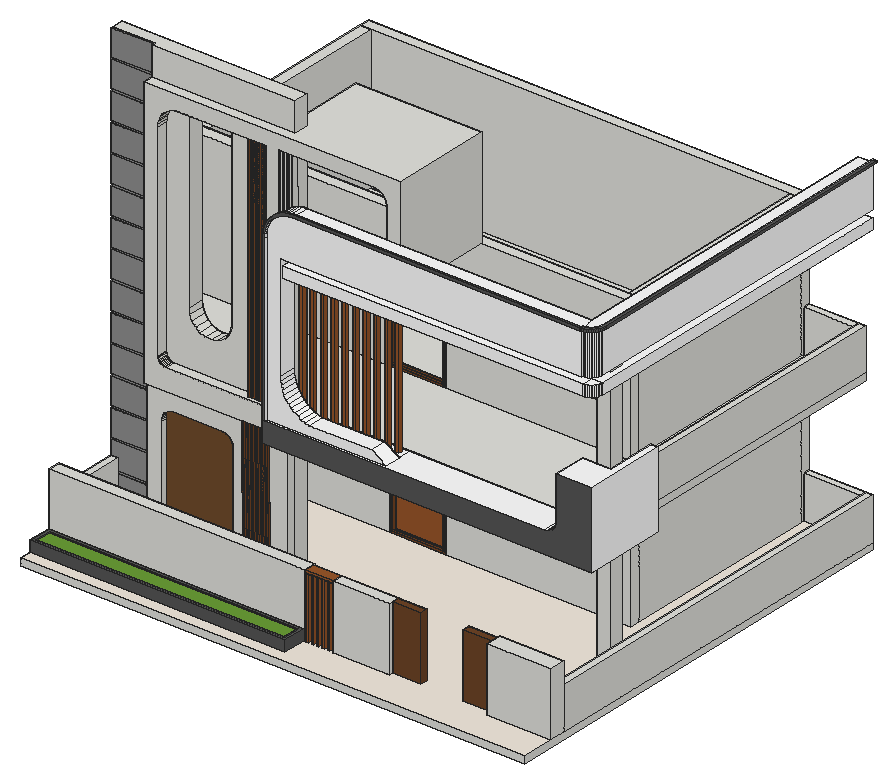
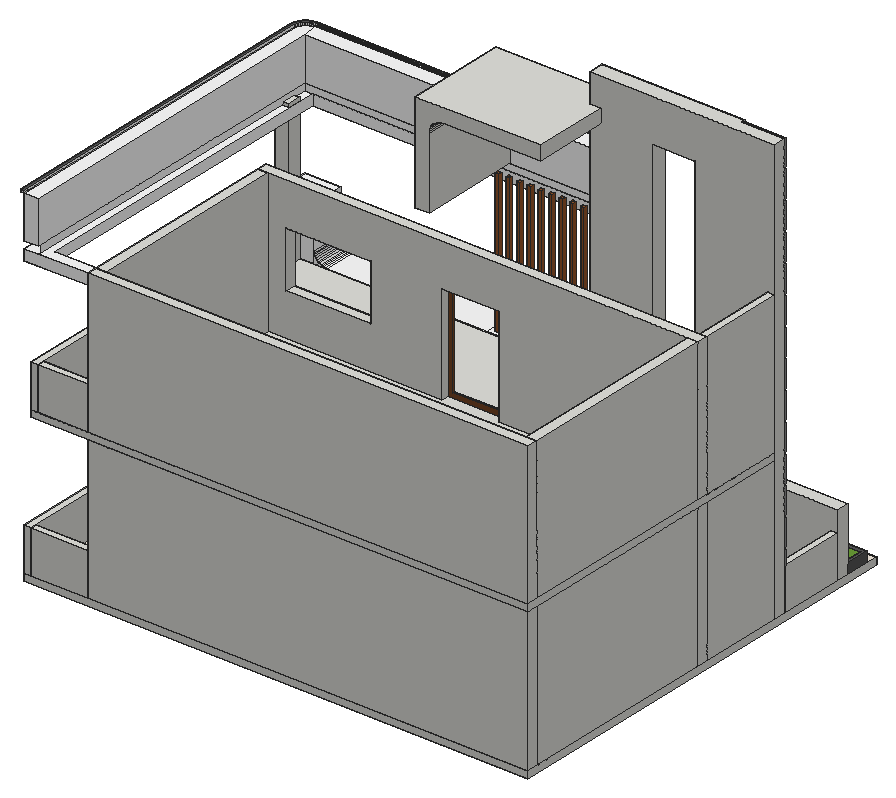
# SketchUp Ruby script. Lengths in inches.
U = 1.inch
M = Sketchup.active_model
def pt(a) = Geom::Point3d.new(a.map { |v| v * U })
def face(e, loops, mat)
  f = e.add_face(loops[0].map { |a| pt(a) })
  loops[1..].each { |l| e.add_face(l.map { |a| pt(a) }).erase! }
  f.material = f.back_material = mat if mat
  f
end
# faces: each face lists its corners as indices into pts; further lists are holes
def faces(e, pts, list, mat = nil) = list.each { |f| face(e, (f[0].is_a?(Array) ? f : [f]).map { |l| l.map { |i| pts[i] } }, mat) }
# xy, xz, yz: faces in a plane at the given z, y or x. An outline is a flat list of corners, or four numbers for a rectangle; further outlines are holes
def ring(l) = l.size == 4 ? [[l[0], l[1]], [l[2], l[1]], [l[2], l[3]], [l[0], l[3]]] : l.each_slice(2).to_a
def flat(e, list, mat, &to3) = list.each { |f| face(e, (f[0].is_a?(Array) ? f : [f]).map { |l| ring(l).map { |u, v| to3.(u, v) } }, mat) }
def xy(e, z, list, mat = nil) = flat(e, list, mat) { |x, y| [x, y, z] }
def xz(e, y, list, mat = nil) = flat(e, list, mat) { |x, z| [x, y, z] }
def yz(e, x, list, mat = nil) = flat(e, list, mat) { |y, z| [x, y, z] }
def lines(e, pts, list) = list.each { |a, b| e.add_line(pt(pts[a]), pt(pts[b])) }
# prism: a flat outline (further loops are holes) pulled along v
def prism(e, loops, v, mat = nil)
  f = face(e, loops, mat); d = Geom::Vector3d.new(v.map { |x| x * U })
  f.pushpull(f.normal.samedirection?(d) ? d.length : -d.length)
end
def box(e, o, s, mat = nil) = prism(e, [[o, [o[0] + s[0], o[1], o[2]], [o[0] + s[0], o[1] + s[1], o[2]], [o[0], o[1] + s[1], o[2]]]], [0, 0, s[2]], mat)
def at(x, y, z, deg = 0) = Geom::Transformation.translation(pt([x, y, z])) * Geom::Transformation.rotation(ORIGIN, Z_AXIS, deg.degrees)
def axes(o, x, y, z) = Geom::Transformation.new([*x, 0, *y, 0, *z, 0, *pt(o).to_a, 1])
def part(name) = M.definitions.add(name)
# library, detail: a bought-in or finely detailed component or shape, given as its bounding box
def library(name, o, s) = part(name).tap { |d| box(d.entities, o, s) }
def detail(e, o, s) = box(e.add_group.entities, o, s)
def put(e, d, t, mat = nil) = e.add_instance(d, t).tap { |i| i.material = mat if mat }
def group(e, t, mat = nil) = e.add_group.tap { |g| g.transformation = t; g.material = mat if mat }.entities
root = M.entities
M.materials.add("[Aluminum]").color = [179, 179, 179]
M.materials.add("[Color M00]").color = [255, 255, 255]
M.materials.add("[Color M04]").color = [142, 142, 142]
M.materials.add("[Color M06]").color = [86, 86, 86]
M.materials.add("[Color M09]").color = [0, 0, 0]
M.materials.add("[Field Rectangle Tile]").color = [242, 233, 221]
M.materials.add("[Grass Dark Green]").color = [106, 157, 55]
M.materials.add("[Translucent Glass Gray]").color = [128, 128, 128]
M.materials["[Translucent Glass Gray]"].alpha = 0.5
M.materials.add("[Wood Board Cork]").color = [181, 169, 96]
M.materials.add("[Wood Cherry Original]").color = [152, 86, 42]
M.materials.add("[Wood Fence with Lattice]").color = [109, 68, 39]
M.materials.add("[Wood Floor]").color = [112, 76, 44]
M.materials.add("[Wood Veneer 01]").color = [120, 70, 37]
c1 = part("Group\#60")
prism(c1.entities,[[[0,3,0.02],[1,3,0.02],[1,2,0],[0,2,0]]],[0.01,-2,107.98])
c2 = part("Group\#7")
xy(c2.entities,0,[[0,0,48,3]])
xy(c2.entities,1.44,[[1.44,0,46.56,0.5]])
xy(c2.entities,2,[[2,0,46,0.5]])
xy(c2.entities,3.15,[[3.15,0,44.85,1.375]])
xy(c2.entities,4,[[4,1.375,44,3]])
xy(c2.entities,80,[[4,1.375,44,3]])
xy(c2.entities,80.85,[[3.15,0,44.85,1.375]])
xy(c2.entities,82,[[2,0,46,0.5]])
xy(c2.entities,82.56,[[1.44,0,46.56,0.5]])
xy(c2.entities,84,[[0,0,48,3]])
xz(c2.entities,0,[[[0,0,48,84],[1.44,1.44,46.56,82.56]],[[2,2,46,82],[3.15,3.15,44.85,80.85]]])
xz(c2.entities,0.5,[[[1.44,1.44,46.56,82.56],[2,2,46,82]]])
xz(c2.entities,1.375,[[[3.15,3.15,44.85,80.85],[4,4,44,80]]])
xz(c2.entities,3,[[[0,0,48,84],[4,4,44,80]]])
yz(c2.entities,0,[[0,0,3,84]])
yz(c2.entities,1.44,[[0,1.44,0.5,82.56]])
yz(c2.entities,2,[[0,2,0.5,82]])
yz(c2.entities,3.15,[[0,3.15,1.375,80.85]])
yz(c2.entities,4,[[1.375,4,3,80]])
yz(c2.entities,44,[[1.375,4,3,80]])
yz(c2.entities,44.85,[[0,3.15,1.375,80.85]])
yz(c2.entities,46,[[0,2,0.5,82]])
yz(c2.entities,46.56,[[0,1.44,0.5,82.56]])
yz(c2.entities,48,[[0,0,3,84]])
c3 = part("Group\#12")
box(c3.entities,[0,0,0],[9,171,120])
c4 = part("Group\#8")
box(c4.entities,[0,-2,0],[40,2,76])
c5 = part("Group\#13")
prism(c5.entities,[[[1.25,1.5,24.92],[1.25,1.5,26.5625],[1.25,0,26.5625],[1.25,0,0],[1.25,1.5,0],[1.25,1.5,1.64],[1.25,0.64,1.64],[1.25,0.64,24.92]]],[-1.25,0,0])
c6 = part("Group\#3")
prism(c6.entities,[[[0,3,0],[0,3,48],[72,3,48],[72,3,0]],[[24,3,3],[24,3,45],[3,3,45],[3,3,3]],[[69,3,45],[48,3,45],[48,3,3],[69,3,3]],[[45,3,3],[45,3,45],[27,3,45],[27,3,3]]],[0,-3,0])
c7 = part("Group\#4")
xz(c7.entities,0,[[0,0,21,42]])
c8 = part("Group\#5")
xz(c8.entities,0,[[0,0,18,42]])
c9 = part("Group\#6")
xz(c9.entities,0,[[0,0,21,42]])
c10 = part("Group\#37")
box(c10.entities,[0,0,0],[3,3,120])
xy(root,132,[[150.78,85.84,150.98,85.85,151.19,85.87,151.39,85.91,151.6,85.96,151.79,86.02,151.99,86.09,152.17,86.18,152.36,86.28,152.53,86.39,150.16,85.9,150.36,85.86]])
xz(root,85.88,[[148.16,114,150.16,132,148.16,132]])
p = [[121.5,94.33,132],[54.63,94.33,132],[53.91,94.33,132.04],[53.2,94.33,132.16],[52.5,94.33,132.35],[51.84,94.33,132.62],
  [51.2,94.33,132.96]]
lines(root,p,[[0,1],[1,2],[2,3],[3,4],[4,5],[5,6]])
g1 = group(root,at(-107.28,-0.61,0))
xy(g1,0,[[107.28,0.61,534,369]])
xy(g1,6,[[107.28,0.61,534,369]],"[Field Rectangle Tile]")
xz(g1,0.61,[[107.28,0,534,6]])
xz(g1,369,[[107.28,0,534,6]])
yz(g1,107.28,[[0.61,0,369,6]])
yz(g1,534,[[0.61,0,369,6]])
g2 = group(root,at(36.03,70.42,6))
g3 = group(g2,at(0,0,0))
xy(g3,0,[[120.65,17.125,73.76,17.42,73.79,21.55,12.79,21.93,12.77,17.81,0.11,17.89,0.15,24.67,120.6875,23.91]])
xy(g3,93.02,[[63.85,17.48,23.45,17.74,23.48,21.86,63.88,21.61]])
xy(g3,108,[[120.65,17.125,120.6875,23.91,0.15,24.67,0.11,17.89]])
p = [[12.77,17.81,0],[12.77,17.81,82.34],[12.86,17.81,83.73],[13.13,17.81,85.1],[13.58,17.8,86.43],[14.2,17.8,87.68],
  [14.97,17.79,88.84],[15.9,17.79,89.89],[16.95,17.78,90.81],[18.11,17.77,91.59],[19.36,17.77,92.21],[20.6875,17.76,92.66],
  [22.06,17.75,92.93],[23.45,17.74,93.02],[63.85,17.48,93.02],[65.15,17.48,92.9375],[66.42,17.47,92.6875],[67.65,17.46,92.27],
  [68.81,17.45,91.7],[69.89,17.45,90.98],[70.86,17.44,90.12],[71.72,17.43,89.15],[72.4375,17.43,88.07],[73.01,17.43,86.91],
  [73.43,17.42,85.68],[73.68,17.42,84.41],[73.76,17.42,83.11],[73.76,17.42,0],[120.65,17.125,0],[120.65,17.125,108],
  [0.11,17.89,108],[0.11,17.89,0],[120.6875,23.91,0],[120.6875,23.91,108],[73.79,21.55,83.11],[73.79,21.55,0],
  [12.79,21.93,0],[12.79,21.93,82.34],[0.15,24.67,108],[0.15,24.67,0],[73.71,21.55,84.41],[73.45,21.55,85.68],
  [73.04,21.55,86.91],[72.46,21.55,88.07],[71.74,21.56,89.15],[70.89,21.56,90.12],[69.91,21.57,90.98],[68.84,21.58,91.7],
  [67.67,21.59,92.27],[66.45,21.59,92.6875],[65.17,21.6,92.9375],[63.88,21.61,93.02],[23.48,21.86,93.02],[22.08,21.875,92.93],
  [20.71,21.88,92.66],[19.39,21.89,92.21],[18.14,21.9,91.59],[16.97,21.91,90.81],[15.92,21.91,89.89],[15,21.92,88.84],
  [14.22,21.92,87.68],[13.6,21.93,86.43],[13.16,21.93,85.1],[12.88,21.93,83.73]]
faces(g3,p,[[0,1,2,3,4,5,6,7,8,9,10,11,12,13,14,15,16,17,18,19,20,21,22,23,24,25,26,27,28,29,30,31],[32,33,29,28],[27,26,34,35],[1,0,36,37],[38,39,31,30],[39,38,33,32],[2,1,37,63],[26,25,40,34],
  [3,2,63,62],[25,24,41,40],[4,3,62,61],[24,23,42,41],[5,4,61,60],[23,22,43,42],[6,5,60,59],[22,21,44,43],
  [7,6,59,58],[21,20,45,44],[8,7,58,57],[20,19,46,45],[9,8,57,56],[19,18,47,46],[10,9,56,55],[18,17,48,47],
  [11,10,55,54],[17,16,49,48],[16,15,50,49],[12,11,54,53],[15,14,51,50],[13,12,53,52]])
faces(g3,p,[[35,34,40,41,42,43,44,45,46,47,48,49,50,51,52,53,54,55,56,57,58,59,60,61,62,63,37,36]],"[Wood Floor]")
put(g3,c1,at(83.21,14.3125,0),"[Wood Veneer 01]")
put(g3,c1,at(84.21,14.3125,0),"[Wood Veneer 01]")
put(g3,c1,at(87.21,14.3125,0),"[Wood Veneer 01]")
put(g3,c1,at(88.21,14.32,0),"[Wood Veneer 01]")
put(g3,c1,at(91.21,14.3125,0),"[Wood Veneer 01]")
put(g3,c1,at(92.21,14.3125,0),"[Wood Veneer 01]")
g4 = group(g3,at(95.21,14.3125,0),"[Wood Veneer 01]")
prism(g4,[[[0,3,0.02],[1,3,0.02],[1,2,0],[0,2,0]]],[0.01,-2,107.98])
g5 = group(g3,at(96.21,14.3125,0),"[Wood Veneer 01]")
prism(g5,[[[0,3,0.02],[1,3,0.02],[1,2,0],[0,2,0]]],[0.01,-2,107.98])
put(g3,c1,at(100.21,14.3125,0),"[Wood Veneer 01]")
put(g3,c1,at(99.21,14.3125,0),"[Wood Veneer 01]")
put(g3,c1,at(104.21,14.3125,0),"[Wood Veneer 01]")
put(g3,c1,at(103.21,14.3125,0),"[Wood Veneer 01]")
g6 = group(root,at(217.625,30.15,6),"[Wood Cherry Original]")
box(g6,[0,0,0],[2.02,9.01,52])
g7 = group(root,at(222.125,30.15,6),"[Wood Cherry Original]")
box(g7,[0,0,0],[2.02,9.01,52])
g8 = group(root,at(226.625,30.15,6),"[Wood Cherry Original]")
box(g8,[0,0,0],[2.02,9.01,52])
g9 = group(root,at(231.125,30.15,6),"[Wood Cherry Original]")
box(g9,[0,0,0],[2.02,9.01,52])
g10 = group(root,at(235.625,30.15,6),"[Wood Cherry Original]")
box(g10,[0,0,0],[2.02,9.01,52])
g11 = group(root,at(-107.28,179.39,6))
prism(g11,[[[480,9,0],[324,9,0],[324,9,84],[276,9,84],[276,9,0],[107.28,9,0],[107.28,9,120],[480,9,120]],[[384,9,84],[384,9,36],[456,9,36],[456,9,84]]],[0,-9,0])
put(root,c2,at(168.72,179.39,6),"[Wood Veneer 01]")
g12 = group(root,at(-107.28,359.39,6))
box(g12,[107.28,0,0],[372.72,9,120])
g13 = group(root,at(363.72,188.39,6))
box(g13,[0,0,0],[9,171,120])
put(root,c3,at(0,188.39,6))
g14 = group(root,at(408.72,98.39,-8.1875))
box(g14,[0,0,14.1875],[12,12,108])
g15 = group(root,at(-17.28,98.39,6))
xy(g15,0,[[53.28,-4.05,53.28,-1.05,17.28,-1.05,17.28,9,174,9,174,-4.05]])
xy(g15,324,[[84.78,-4.05,120.78,9]])
xy(g15,360,[[53.28,-4.05,174,-4.05,174,9,17.28,9,17.28,-1.05,53.28,-1.05]])
xz(g15,-4.05,[[[53.28,0,174,360],[102.78,153.9,98.12,154.51,93.78,156.31,90.05,159.17,87.19,162.9,85.39,167.24,84.78,171.9,84.78,324,120.78,324,120.78,171.9,120.17,167.24,118.37,162.9,115.51,159.17,111.78,156.31,107.4375,154.51]]])
xz(g15,-1.05,[[17.28,0,53.28,360]])
xz(g15,9,[[[17.28,0,174,360],[102.78,153.9,107.4375,154.51,111.78,156.31,115.51,159.17,118.37,162.9,120.17,167.24,120.78,171.9,120.78,324,84.78,324,84.78,171.9,85.39,167.24,87.19,162.9,90.05,159.17,93.78,156.31,98.12,154.51]]])
yz(g15,17.28,[[-1.05,0,9,360]])
yz(g15,53.28,[[-4.05,0,-1.05,360]])
yz(g15,84.78,[[-4.05,171.9,9,324]])
yz(g15,120.78,[[-4.05,171.9,9,324]])
yz(g15,174,[[-4.05,0,9,360]])
p = [[98.12,9,154.51],[98.12,-4.05,154.51],[102.78,-4.05,153.9],[102.78,9,153.9],[107.4375,-4.05,154.51],[107.4375,9,154.51],
  [93.78,9,156.31],[93.78,-4.05,156.31],[111.78,-4.05,156.31],[111.78,9,156.31],[90.05,9,159.17],[90.05,-4.05,159.17],
  [115.51,-4.05,159.17],[115.51,9,159.17],[87.19,9,162.9],[87.19,-4.05,162.9],[118.37,-4.05,162.9],[118.37,9,162.9],
  [85.39,9,167.24],[85.39,-4.05,167.24],[120.17,-4.05,167.24],[120.17,9,167.24],[84.78,9,171.9],[84.78,-4.05,171.9],
  [120.78,-4.05,171.9],[120.78,9,171.9],[53.46,-3.29,108],[174.03,-3.29,108]]
faces(g15,p,[[0,1,2,3],[3,2,4,5],[6,7,1,0],[5,4,8,9],[10,11,7,6],[9,8,12,13],[14,15,11,10],[13,12,16,17],
  [18,19,15,14],[17,16,20,21],[22,23,19,18],[21,20,24,25]])
lines(g15,p,[[26,27]])
g16 = group(root,at(0,95.83,6),"[Color M04]")
prism(g16,[[[36,1.5,0],[36,1.5,360],[36,0,360],[36,0,338],[36,0.5,338],[36,0.5,336],[36,0,336],[36,0,314],[36,0.5,314],[36,0.5,312],[36,0,312],[36,0,290],[36,0.5,290],[36,0.5,288],[36,0,288],[36,0,266],[36,0.5,266],[36,0.5,264],[36,0,264],[36,0,242],[36,0.5,242],[36,0.5,240],[36,0,240],[36,0,218],[36,0.5,218],[36,0.5,216],[36,0,216],[36,0,194],[36,0.5,194],[36,0.5,192],[36,0,192],[36,0,170],[36,0.5,170],[36,0.5,168],[36,0,168],[36,0,146],[36,0.5,146],[36,0.5,144],[36,0,144],[36,0,122],[36,0.5,122],[36,0.5,120],[36,0,120],[36,0,98],[36,0.5,98],[36,0.5,96],[36,0,96],[36,0,74],[36,0.5,74],[36,0.5,72],[36,0,72],[36,0,50],[36,0.5,50],[36,0.5,48],[36,0,48],[36,0,26],[36,0.5,26],[36,0.5,24],[36,0,24],[36,0,0]]],[-36,0,0])
g17 = group(root,at(0,107.39,6))
box(g17,[0,0,0],[6,72,120])
g18 = group(root,at(0,30.17,6))
box(g18,[0,0,0],[216.72,10.37,54])
g19 = group(root,at(348.72,29.18,6),"[Wood Fence with Lattice]")
box(g19,[0,3,0],[24,6.15,54])
g20 = group(root,at(288.72,29.56,6),"[Wood Fence with Lattice]")
box(g20,[0,3,0],[24,6.15,54])
g21 = group(root,at(372.72,27.34,6))
box(g21,[0,0,0],[54,13.5,54])
g22 = group(root,at(420.72,40.84,6))
box(g22,[0,0,0],[6,327.55,36])
g23 = group(root,at(372.72,362.39,6))
box(g23,[0,0,0],[48,6,36])
g24 = group(root,at(240.72,29.71,6))
box(g24,[0,0,0],[48,9.3,54])
g25 = group(root,at(0,10.04,6),"[Color M06]")
xy(g25,0,[[0,0,215.875,20.125]])
xy(g25,8.375,[[2.92,2.92,212.95,17.2]],"[Grass Dark Green]")
xy(g25,9.0625,[[[0,0,215.875,20.125],[2.92,2.92,212.95,17.2]]])
xz(g25,0,[[0,0,215.875,9.0625]],"[Color M06]")
xz(g25,2.92,[[2.92,8.375,212.95,9.0625]])
xz(g25,17.2,[[2.92,8.375,212.95,9.0625]])
xz(g25,20.125,[[0,0,215.875,9.0625]])
yz(g25,0,[[0,0,20.125,9.0625]])
yz(g25,2.92,[[2.92,8.375,17.2,9.0625]])
yz(g25,212.95,[[2.92,8.375,17.2,9.0625]])
yz(g25,215.875,[[0,0,20.125,9.0625]])
g26 = group(root,at(0,40.54,6))
box(g26,[0,0,0],[6,55.29,36])
put(root,c4,at(172.72,182.76,10),"[Wood Cherry Original]")
put(root,c5,at(207.62,179.26,37.75),"[Aluminum]")
put(root,c6,at(276.72,181.39,42),"[Color M09]")
put(root,c7,at(324.72,181.39,45),"[Translucent Glass Gray]")
put(root,c8,at(303.72,181.39,45),"[Translucent Glass Gray]")
put(root,c9,at(279.72,181.39,45),"[Translucent Glass Gray]")
g27 = group(root,at(216.72,30.15,58),"[Wood Cherry Original]")
box(g27,[0,0,0],[24,9.01,2])
g28 = group(root,at(156.72,177.39,90),"[Wood Board Cork]")
prism(g28,[[[-21.9375,2,0],[216,2,0],[216,11,0],[218,11,0],[218,0,0],[-21.9375,0,0]]],[0,0,12])
g29 = group(root,at(36,85.33,114))
xy(g29,0,[[0.06,0,0,12,120.72,12.59,120.75,7.34,120.75,7.33,120.7,6.46,120.53,5.59,120.25,4.75,119.86,3.96,119.375,3.22,118.8,2.56,118.13,1.97,117.4,1.48,116.61,1.08,115.78,0.79,114.91,0.62,114.03,0.55]])
xy(g29,18,[[18.67,0.09,102.78,0.5,102.72,12.5,18.62,12.09]])
xy(g29,144,[[204.78,1,204.36,86.74,216.36,86.8,216.78,1.05]])
xy(g29,216,[[29.88,0.14,29.82,12.14,102.72,12.5,102.78,0.5],[102.78,0.5,102.72,12.5,110.85,12.54,110.49,86.29,193.29,86.69,193.71,0.94,114.02,0.55],[102.78,0.5,114.02,0.55,114.91,0.62,115.77,0.79,116.61,1.08,117.4,1.48,118.13,1.97,118.79,2.56,119.37,3.22,119.86,3.96,120.24,4.75,120.52,5.59,120.69,6.46,120.74,7.34,120.72,12.59,110.85,12.54,102.72,12.5]])
xy(g29,228,[[0.06,0,216.78,1.05,216.36,86.8,110.49,86.29,110.85,12.54,0,12]])
p = [[0,12,228],[0,12,0],[0.06,0,0],[0.06,0,228],[114.03,0.55,0],[114.02,0.55,216],
  [193.71,0.94,216],[195.16,0.95,215.91],[196.58,0.96,215.62],[197.95,0.96,215.16],[199.25,0.97,214.52],[200.45,0.97,213.71],
  [201.54,0.98,212.76],[202.49,0.98,211.67],[203.3,0.99,210.47],[203.9375,0.99,209.17],[204.4,0.99,207.8],[204.69,0.99,206.375],
  [204.78,1,204.93],[204.78,1,144],[216.78,1.05,144],[216.78,1.05,228],[102.78,0.5,18],[18.67,0.09,18],
  [17.8125,0.09,18.06],[16.96,0.08,18.23],[16.14,0.08,18.5],[15.37,0.07,18.89],[14.65,0.07,19.37],[14,0.07,19.9375],
  [13.43,0.06,20.59],[12.94,0.0625,21.31],[12.5625,0.0625,22.09],[12.28,0.06,22.9],[12.11,0.06,23.75],[12.06,0.06,24.62],
  [12.06,0.06,198.18],[12.21,0.06,200.5],[12.67,0.0625,202.79],[13.41,0.06,205],[14.45,0.07,207.09],[15.74,0.08,209.03],
  [17.28,0.08,210.78],[19.03,0.09,212.32],[20.97,0.1,213.61],[23.06,0.11,214.64],[25.27,0.12,215.39],[27.55,0.13,215.85],
  [29.88,0.14,216],[102.78,0.5,216],[114.91,0.62,0],[114.91,0.62,216],[115.78,0.79,0],[115.77,0.79,216],
  [116.61,1.08,0],[116.61,1.08,216],[117.4,1.48,0],[117.4,1.48,216],[118.13,1.97,0],[118.13,1.97,216],
  [118.8,2.56,0],[118.79,2.56,216],[119.375,3.22,0],[119.37,3.22,216],[119.86,3.96,0],[119.86,3.96,216],
  [120.25,4.75,0],[120.24,4.75,216],[120.53,5.59,0],[120.52,5.59,216],[120.7,6.46,0],[120.69,6.46,216],
  [120.75,7.34,0],[120.74,7.34,216],[120.75,7.33,0],[120.72,12.59,0],[120.72,12.59,216],[110.85,12.54,228],
  [110.85,12.54,216],[102.72,12.5,18],[102.72,12.5,216],[29.82,12.14,216],[27.5,12.13,215.85],[25.21,12.12,215.39],
  [23,12.11,214.64],[20.91,12.1,213.61],[18.97,12.09,212.32],[17.22,12.08,210.78],[15.68,12.08,209.03],[14.39,12.07,207.09],
  [13.36,12.06,205],[12.61,12.0625,202.79],[12.15,12.06,200.5],[12,12.06,198.18],[12,12.06,24.62],[12,12.06,18],
  [18.62,12.09,18],[17.75,12.09,18.06],[12.06,12.06,23.75],[12.23,12.06,22.9],[12.5,12.0625,22.09],[12.89,12.0625,21.31],
  [13.37,12.06,20.59],[13.9375,12.07,19.9375],[14.59,12.07,19.37],[15.31,12.07,18.89],[16.08,12.08,18.5],[16.9,12.08,18.23],
  [204.36,86.74,204.93],[204.36,86.74,144],[216.36,86.8,144],[216.36,86.8,228],[193.29,86.69,216],[110.49,86.29,216],
  [110.49,86.29,228],[204.27,86.74,206.375],[203.99,86.74,207.8],[203.52,86.74,209.17],[202.88,86.74,210.47],[202.08,86.73,211.67],
  [201.12,86.73,212.76],[200.03,86.72,213.71],[198.83,86.72,214.52],[197.53,86.71,215.16],[196.16,86.7,215.62],[194.74,86.7,215.91],
  [12.06,0.06,18]]
faces(g29,p,[[0,1,2,3],[[4,5,6,7,8,9,10,11,12,13,14,15,16,17,18,19,20,21,3,2],[22,23,24,25,26,27,28,29,30,31,32,33,34,35,36,37,38,39,40,41,42,43,44,45,46,47,48,49]],[50,51,5,4],[52,53,51,50],[54,55,53,52],[56,57,55,54],[58,59,57,56],[60,61,59,58],
  [62,63,61,60],[64,65,63,62],[66,67,65,64],[68,69,67,66],[70,71,69,68],[72,73,71,70,74],[73,72,75,76],[[0,77,78,76,75,1],[79,80,81,82,83,84,85,86,87,88,89,90,91,92,93,94,95,96]],
  [24,23,96,97],[79,22,49,80],[97,96,95,94,98,99,100,101,102,103,104,105,106,107],[25,24,97,107],[26,25,107,106],[27,26,106,105],[28,27,105,104],[29,28,104,103],
  [30,29,103,102],[31,30,102,101],[32,31,101,100],[33,32,100,99],[34,33,99,98],[35,34,98,94],[36,35,94,93],[18,108,109,19],
  [20,110,111,21],[112,113,114,111,110,109,108,115,116,117,118,119,120,121,122,123,124,125],[93,92,37,36],[92,91,38,37],[91,90,39,38],[17,115,108,18],[90,89,40,39],[16,116,115,17],
  [89,88,41,40],[15,117,116,16],[88,87,42,41],[14,118,117,15],[13,119,118,14],[87,86,43,42],[12,120,119,13],[86,85,44,43],
  [11,121,120,12],[85,84,45,44],[10,122,121,11],[9,123,122,10],[84,83,46,45],[8,124,123,9],[83,82,47,46],[7,125,124,8],
  [82,81,48,47],[6,112,125,7],[78,77,114,113]])
lines(g29,p,[[126,95]])
detail(g29,[130.83,15.11,215.5],[47.25,34.81,0.5])
g30 = group(root,at(150.16,73.55,132),"[Color M00]")
xy(g30,-18,[[-2,-3.07,-2,24.84,270.5625,24.84,270.5625,67.34,276.5625,67.34,276.5625,-3.07]],"[Color M06]")
xy(g30,0,[[0,-3.07,236.39,-3.07,236.39,24.84,101.35,24.84,101.35,-1.07,0,-1.07],[-2,-1.07,0,12.84],[0,-1.07,101.35,12.84],[-2,12.84,101.35,24.84]])
xy(g30,8,[[36,-1.07,88.8125,12.84]])
xy(g30,46.125,[[246.5625,-3.07,276.5625,-3.07,276.5625,67.34,270.5625,67.34,270.5625,24.84,246.5625,24.84]])
xy(g30,111,[[12,0,12,12.84,257.5625,12.84,257.5625,285.15,222.5625,285.15,222.5625,294.84,276,294.84,276,9.74,275.92,8.47,275.69,7.22,275.31,6.01,274.78,4.87,274.12,3.81,273.33,2.85,272.44,2.01,271.45,1.3,270.38,0.74,269.26,0.33,268.09,0.08,266.9,0]])
xy(g30,120,[[12,0,12,12.84,264,12.84,264,9.74,266.9,9.74,266.9,0],[266.9,0,266.9,9.74,276,9.74,275.92,8.47,275.69,7.22,275.31,6.01,274.78,4.87,274.12,3.81,273.33,2.85,272.44,2.01,271.45,1.3,270.38,0.74,269.26,0.33,268.09,0.08],[264,9.74,266.9,12.84],[266.9,9.74,276,9.74,276,294.84,264,294.84,264,12.84,266.9,12.84],[257.5625,12.84,264,12.84,264,294.84,222.5625,294.84,222.5625,285.15,257.5625,285.15]])
xy(g30,126,[[12,-1.07,12,12.84,264,12.84,264,9.74,266.9,9.74,266.9,-1.07],[266.9,0,266.9,9.74,276,9.74,275.92,8.47,275.69,7.22,275.31,6.01,274.78,4.87,274.12,3.81,273.33,2.85,272.44,2.01,271.45,1.3,270.38,0.74,269.26,0.33,268.09,0.08],[264,9.74,266.9,12.84],[266.9,9.74,266.9,12.84,264,12.84,264,294.84,276,294.84,276,9.74]])
xy(g30,162,[[23.56,-3.07,23.56,-1.07,266.9,-1.07,266.9,-3.04,266.42,-3.07],[266.42,-3.07,266.9,-3.04,266.9,-3.07],[23.56,-1.07,266.9,-1.07,266.9,0,264,12.84,23.56,12.84],[266.9,0,268.09,0.08,269.26,0.33,270.38,0.74,271.45,1.3,272.44,2.01,273.33,2.85,274.12,3.81,274.78,4.87,275.31,6.01,275.69,7.22,275.92,8.47,276,9.74,276,294.84,264,294.84,264,12.84]])
xy(g30,164,[[23.56,-3.07,266.9,-1.07],[266.9,-3.04,266.9,0,268.09,0.08,269.26,0.33,270.38,0.74,271.45,1.3,272.44,2.01,273.33,2.85,274.12,3.81,274.78,4.87,275.31,6.01,275.69,7.22,275.92,8.47,276,9.74,276,295.14,279.03,295.14,279.03,9.64,278.93,8.1,278.63,6.48,278.14,4.91,277.45,3.43,276.59,2.04,275.55,0.78,274.37,-0.33,273.04,-1.28,271.61,-2.03,270.09,-2.59,268.51,-2.92]],"[Color M06]")
xz(g30,-3.07,[[-2,-18,276.5625,-18,276.5625,46.125,246.5625,46.125,246.5625,10.17,246.48,8.85,246.22,7.54,245.79,6.28,245.2,5.09,244.46,3.98,243.58,2.98,242.58,2.1,241.48,1.36,240.28,0.77,239.02,0.35,237.72,0.09,236.39,0,-2,0],[-2,0,0,0,0,138.44,0.2,141.52,0.8,144.54,1.79,147.46,3.16,150.22,4.87,152.78,6.9,155.1,9.22,157.13,11.78,158.84,14.54,160.21,17.46,161.2,20.48,161.8,23.56,162,266.9,162,266.9,164,23.56,164,20.22,163.78,16.94,163.13,13.78,162.05,10.78,160.58,8,158.72,5.49,156.51,3.28,154,1.42,151.22,-0.05,148.22,-1.13,145.06,-1.78,141.78,-2,138.44]],"[Color M06]")
xz(g30,-1.07,[[0,0,101.35,0,88.8125,8,36,8,32.7,8.85,29.51,10.07,26.49,11.65,23.67,13.5625,21.08,15.79,18.77,18.29,16.76,21.05,15.08,24.01,13.74,27.15,12.78,30.42,12.2,33.78,12,37.1875,12,126,266.9,126,266.9,162,23.56,162,20.48,161.8,17.46,161.2,14.54,160.21,11.78,158.84,9.22,157.13,6.9,155.1,4.87,152.78,3.16,150.22,1.79,147.46,0.8,144.54,0.2,141.52,0,138.44]])
xz(g30,0,[[12,111,266.9,120]])
xz(g30,12.84,[[0,0,0,138.44,0.2,141.52,0.8,144.54,1.79,147.46,3.16,150.22,4.87,152.78,6.9,155.1,9.22,157.13,11.78,158.84,14.54,160.21,17.46,161.2,20.48,161.8,23.56,162,264,162,264,126,12,126,12,37.1875,12.2,33.78,12.78,30.42,13.74,27.15,15.08,24.01,16.76,21.05,18.77,18.29,21.08,15.79,23.67,13.5625,26.49,11.65,29.51,10.07,32.7,8.85,36,8,88.8125,8,101.35,0],[12,111,257.5625,120],[12,120,264,126]])
xz(g30,24.84,[[-2,-18,101.35,0],[101.35,-18,101.35,0,246.5625,0,246.5625,46.125,270.5625,46.125,270.5625,-18],[236.39,0,237.72,0.09,239.02,0.35,240.28,0.77,241.48,1.36,242.58,2.1,243.58,2.98,244.46,3.98,245.2,5.09,245.79,6.28,246.22,7.54,246.48,8.85,246.5625,10.17,246.5625,0]])
xz(g30,67.34,[[270.5625,-18,276.5625,46.125]])
xz(g30,285.15,[[222.5625,111,257.5625,120]])
xz(g30,294.84,[[222.5625,111,276,120],[264,126,276,162]])
xz(g30,295.14,[[276,162,279.03,164]])
yz(g30,-2,[[-3.07,-18,-1.07,138.44],[-1.07,-18,24.84,0]],"[Color M06]")
yz(g30,0,[[-3.07,0,-1.07,138.44],[-1.07,0,12.84,138.44]])
yz(g30,12,[[-1.07,37.1875,12.84,37.1875,12.84,111,0,111,0,120,12.84,120,12.84,126,-1.07,126],[0,111,12.84,120]])
yz(g30,222.5625,[[285.15,111,294.84,120]])
yz(g30,246.5625,[[-3.07,10.17,24.84,46.125]])
yz(g30,257.5625,[[12.84,111,285.15,120]])
yz(g30,264,[[12.84,120,292.11,126],[12.84,126,294.84,162]])
yz(g30,266.9,[[-1.07,126,0,162],[-3.07,162,-3.04,164],[-3.04,162,-1.07,164],[-1.07,162,0,164]])
yz(g30,270.5625,[[24.84,-18,67.34,0],[24.84,0,67.34,46.125]])
yz(g30,276,[[9.74,111,294.84,120],[9.74,126,294.84,162],[9.74,162,292.11,164],[292.11,162,295.14,164]])
yz(g30,276.5625,[[-3.07,-18,67.34,46.125]])
yz(g30,279.03,[[9.64,162,295.14,164]],"[Color M06]")
p = [[236.39,-3.07,0],[237.72,-3.07,0.09],[237.72,24.84,0.09],[236.39,24.84,0],[101.35,12.84,0],[88.8125,12.84,8],
  [88.8125,-1.07,8],[101.35,-1.07,0],[239.02,-3.07,0.35],[239.02,24.84,0.35],[240.28,-3.07,0.77],[240.28,24.84,0.77],
  [241.48,-3.07,1.36],[241.48,24.84,1.36],[242.58,-3.07,2.1],[242.58,24.84,2.1],[243.58,-3.07,2.98],[243.58,24.84,2.98],
  [244.46,-3.07,3.98],[244.46,24.84,3.98],[245.2,-3.07,5.09],[245.2,24.84,5.09],[245.79,-3.07,6.28],[245.79,24.84,6.28],
  [246.22,-3.07,7.54],[246.22,24.84,7.54],[246.48,-3.07,8.85],[246.48,24.84,8.85],[36,12.84,8],[32.7,12.84,8.85],
  [32.7,-1.07,8.85],[36,-1.07,8],[246.5625,-3.07,10.17],[246.5625,24.84,10.17],[29.51,12.84,10.07],[29.51,-1.07,10.07],
  [26.49,12.84,11.65],[26.49,-1.07,11.65],[23.67,12.84,13.5625],[23.67,-1.07,13.5625],[21.08,12.84,15.79],[21.08,-1.07,15.79],
  [18.77,12.84,18.29],[18.77,-1.07,18.29],[16.76,12.84,21.05],[16.76,-1.07,21.05],[15.08,12.84,24.01],[15.08,-1.07,24.01],
  [13.74,12.84,27.15],[13.74,-1.07,27.15],[12.78,12.84,30.42],[12.78,-1.07,30.42],[12.2,12.84,33.78],[12.2,-1.07,33.78],
  [12,12.84,37.1875],[12,-1.07,37.1875],[268.09,0.08,120],[266.9,0,120],[266.9,0,111],[268.09,0.08,111],
  [269.26,0.33,120],[269.26,0.33,111],[270.38,0.74,120],[270.38,0.74,111],[271.45,1.3,120],[271.45,1.3,111],
  [272.44,2.01,120],[272.44,2.01,111],[273.33,2.85,120],[273.33,2.85,111],[274.12,3.81,120],[274.12,3.81,111],
  [274.78,4.87,120],[274.78,4.87,111],[275.31,6.01,120],[275.31,6.01,111],[275.69,7.22,120],[275.69,7.22,111],
  [275.92,8.47,120],[275.92,8.47,111],[276,9.74,120],[276,9.74,111],[268.09,0.08,162],[266.9,0,162],
  [266.9,0,126],[268.09,0.08,126],[269.26,0.33,162],[269.26,0.33,126],[270.38,0.74,162],[270.38,0.74,126],
  [271.45,1.3,162],[271.45,1.3,126],[272.44,2.01,162],[272.44,2.01,126],[273.33,2.85,162],[273.33,2.85,126],
  [274.12,3.81,162],[274.12,3.81,126],[274.78,4.87,162],[274.78,4.87,126],[275.31,6.01,162],[275.31,6.01,126],
  [275.69,7.22,162],[275.69,7.22,126],[275.92,8.47,162],[275.92,8.47,126],[276,9.74,162],[276,9.74,126],
  [-1.78,-1.07,141.78],[-2,-1.07,138.44],[-2,-3.07,138.44],[-1.78,-3.07,141.78],[0,-1.07,138.44],[0.2,-1.07,141.52],
  [0.2,-3.07,141.52],[0,-3.07,138.44],[0.2,12.84,141.52],[0,12.84,138.44],[0.8,-1.07,144.54],[0.8,-3.07,144.54],
  [0.8,12.84,144.54],[-1.13,-1.07,145.06],[-1.13,-3.07,145.06],[1.79,-1.07,147.46],[1.79,-3.07,147.46],[1.79,12.84,147.46],
  [-0.05,-1.07,148.22],[-0.05,-3.07,148.22],[3.16,-1.07,150.22],[3.16,-3.07,150.22],[3.16,12.84,150.22],[1.42,-1.07,151.22],
  [1.42,-3.07,151.22],[4.87,-1.07,152.78],[4.87,-3.07,152.78],[4.87,12.84,152.78],[3.28,-1.07,154],[3.28,-3.07,154],
  [6.9,-1.07,155.1],[6.9,-3.07,155.1],[6.9,12.84,155.1],[5.49,-1.07,156.51],[5.49,-3.07,156.51],[9.22,-1.07,157.13],
  [9.22,-3.07,157.13],[9.22,12.84,157.13],[8,-1.07,158.72],[8,-3.07,158.72],[11.78,-1.07,158.84],[11.78,-3.07,158.84],
  [11.78,12.84,158.84],[10.78,-1.07,160.58],[10.78,-3.07,160.58],[14.54,-1.07,160.21],[14.54,-3.07,160.21],[14.54,12.84,160.21],
  [17.46,-1.07,161.2],[17.46,-3.07,161.2],[17.46,12.84,161.2],[13.78,-1.07,162.05],[13.78,-3.07,162.05],[20.48,-1.07,161.8],
  [20.48,-3.07,161.8],[20.48,12.84,161.8],[23.56,-1.07,162],[23.56,-3.07,162],[23.56,12.84,162],[268.51,-2.92,162],
  [266.9,-3.04,162],[266.9,-3.04,164],[268.51,-2.92,164],[270.09,-2.59,162],[270.09,-2.59,164],[271.61,-2.03,162],
  [271.61,-2.03,164],[273.04,-1.28,162],[273.04,-1.28,164],[274.37,-0.33,162],[274.37,-0.33,164],[275.55,0.78,162],
  [275.55,0.78,164],[268.09,0.08,164],[266.9,0,164],[269.26,0.33,164],[270.38,0.74,164],[271.45,1.3,164],
  [276.59,2.04,162],[276.59,2.04,164],[272.44,2.01,164],[273.33,2.85,164],[277.45,3.43,162],[277.45,3.43,164],
  [274.12,3.81,164],[278.14,4.91,162],[278.14,4.91,164],[274.78,4.87,164],[275.31,6.01,164],[278.63,6.48,162],
  [278.63,6.48,164],[275.69,7.22,164],[278.93,8.1,162],[278.93,8.1,164],[275.92,8.47,164],[279.03,9.64,162],
  [279.03,9.64,164],[276,9.74,164],[16.94,-1.07,163.13],[16.94,-3.07,163.13],[20.22,-1.07,163.78],[20.22,-3.07,163.78],
  [23.56,-1.07,164],[23.56,-3.07,164],[260.97,12.84,162],[260.97,12.5,162],[101.35,-1.07,-18],[246.5625,-3.07,0],
  [246.5625,24.84,0]]
faces(g30,p,[[0,1,2,3],[4,5,6,7],[1,8,9,2],[8,10,11,9],[10,12,13,11],[12,14,15,13],[14,16,17,15],[16,18,19,17],
  [18,20,21,19],[20,22,23,21],[22,24,25,23],[24,26,27,25],[28,29,30,31],[26,32,33,27],[29,34,35,30],[34,36,37,35],
  [36,38,39,37],[38,40,41,39],[40,42,43,41],[42,44,45,43],[44,46,47,45],[46,48,49,47],[48,50,51,49],[50,52,53,51],
  [52,54,55,53],[56,57,58,59],[60,56,59,61],[62,60,61,63],[64,62,63,65],[66,64,65,67],[68,66,67,69],[70,68,69,71],
  [72,70,71,73],[74,72,73,75],[76,74,75,77],[78,76,77,79],[80,78,79,81],[82,83,84,85],[86,82,85,87],[88,86,87,89],
  [90,88,89,91],[92,90,91,93],[94,92,93,95],[96,94,95,97],[98,96,97,99],[100,98,99,101],[102,100,101,103],[104,102,103,105],
  [106,104,105,107],[112,113,114,115],[116,117,112,113],[113,118,119,114],[120,116,113,118],[118,123,124,119],[125,120,118,123],[123,128,129,124],
  [130,125,123,128],[128,133,134,129],[135,130,128,133],[133,138,139,134],[140,135,133,138],[138,143,144,139],[145,140,138,143],[143,148,149,144],
  [150,145,143,148],[148,153,154,149],[155,150,148,153],[153,156,157,154],[158,155,153,156],[156,161,162,157],[163,158,156,161],[161,164,165,162],
  [166,163,161,164],[83,82,181,182],[82,86,183,181],[86,88,184,183],[88,90,185,184],[90,92,188,185],[92,94,189,188],[94,96,192,189],
  [96,98,195,192],[98,100,196,195],[100,102,199,196],[102,104,202,199],[104,106,205,202]])
faces(g30,p,[[108,109,110,111],[121,108,111,122],[126,121,122,127],[131,126,127,132],[136,131,132,137],[141,136,137,142],[146,141,142,147],[151,146,147,152],
  [159,151,152,160],[167,168,169,170],[171,167,170,172],[173,171,172,174],[175,173,174,176],[177,175,176,178],[179,177,178,180],[186,179,180,187],
  [190,186,187,191],[193,190,191,194],[197,193,194,198],[200,197,198,201],[203,200,201,204],[206,159,160,207],[208,206,207,209],[210,208,209,211]],"[Color M06]")
lines(g30,p,[[212,213],[7,214],[215,216]])
g31 = group(root,at(-17.28,179.39,126))
prism(g31,[[[174,-72,0],[17.28,-72,0],[17.28,189,0],[438,189,0],[438,-81,0],[174,-81,0]]],[0,0,6])
put(root,c10,at(162.94,91.31,132),"[Wood Cherry Original]")
put(root,c10,at(171.94,91.31,132),"[Wood Cherry Original]")
put(root,c10,at(180.94,91.31,132),"[Wood Cherry Original]")
put(root,c10,at(189.94,91.31,132),"[Wood Cherry Original]")
put(root,c10,at(198.94,91.31,132),"[Wood Cherry Original]")
put(root,c10,at(207.94,91.31,132),"[Wood Cherry Original]")
put(root,c10,at(216.94,91.31,132),"[Wood Cherry Original]")
put(root,c10,at(225.94,91.31,132),"[Wood Cherry Original]")
put(root,c10,at(234.94,91.31,132),"[Wood Cherry Original]")
put(root,c10,at(243.94,91.31,132),"[Wood Cherry Original]")
put(root,c2,at(168.72,179.39,132),"[Wood Veneer 01]")
put(root,c3,at(0,188.39,132))
g32 = group(root,at(-107.28,179.39,132))
prism(g32,[[[480,9,0],[324,9,0],[324,9,84],[276,9,84],[276,9,0],[107.28,9,0],[107.28,9,120],[480,9,120]],[[384,9,84],[384,9,36],[456,9,36],[456,9,84]]],[0,-9,0])
g33 = group(root,at(-107.28,359.39,132))
box(g33,[107.28,0,0],[372.72,9,120])
g34 = group(root,at(363.72,188.39,132))
box(g34,[0,0,0],[9,171,120])
g35 = group(root,at(414.72,110.39,132))
box(g35,[0,0,0],[6,258,36])
g36 = group(root,at(372.72,362.39,132))
box(g36,[0,0,0],[42,6,36])
g37 = group(root,at(0,107.39,132))
box(g37,[0,0,0],[6,72,120])
g38 = group(root,at(408.72,98.39,132))
xy(g38,0,[[0,0,12,12]])
xy(g38,122.1875,[[0,0,12,12]])
xz(g38,0,[[0,0,12,111],[0,111,12,122.1875]])
xz(g38,12,[[0,0,12,122.1875]])
yz(g38,0,[[0,0,12,122.1875]])
yz(g38,12,[[0,0,12,111],[0,111,12,122.1875]])
g39 = group(root,at(121.5,89.33,132),"[Wood Veneer 01]")
xy(g39,0,[[0,-0.5,0,8,18,8,18,0,17,0,17,0.5,16,0.5,16,0,13,0,13,0.5,10,0.5,10,0,7,0,7,0.5,6,0.5,6,0,3,0,3,0.5,1,0.5,1,-0.5],[16,0.375,17,0.5]])
xy(g39,198,[[0,-0.5,1,-0.5,1,0.5,3,0.5,3,0,6,0,6,0.5,7,0.5,7,0,10,0,10,0.5,13,0.5,13,0,16,0,16,0.5,17,0.5,17,0,18,0,18,8,0,8],[16,0.375,17,0.5],[16,0.375,17,0.5]])
xz(g39,-0.5,[[0,0,1,198]])
xz(g39,0,[[3,0,4,198],[4,0,5,198],[5,0,6,198],[7,0,8,198],[8,0,9,198],
  [9,0,10,198],[13,0,14,198],[14,0,15,198],[15,0,16,198],[17,0,18,198]])
xz(g39,0.375,[[16,0,17,198]])
xz(g39,0.5,[[1,0,2,198],[2,0,3,198],[6,0,7,198],[10,0,11,198],[11,0,12,198],
  [12,0,13,198],[16,0,17,198]])
xz(g39,8,[[0,0,18,198]])
yz(g39,0,[[-0.5,0,8,198]])
yz(g39,1,[[-0.5,0,0.5,198]])
yz(g39,3,[[0,0,0.5,198]])
yz(g39,6,[[0,0,0.5,198]])
yz(g39,7,[[0,0,0.5,198]])
yz(g39,10,[[0,0,0.5,198]])
yz(g39,13,[[0,0,0.5,198]])
yz(g39,16,[[0,0,0.375,198],[0.375,0,0.5,198]])
yz(g39,17,[[0,0,0.375,198],[0.375,0,0.5,198]])
yz(g39,18,[[0,0,8,198]])
